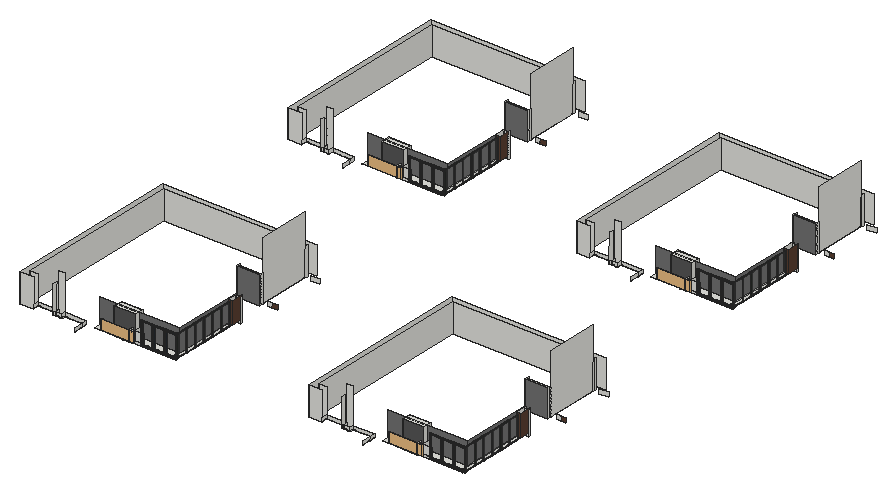
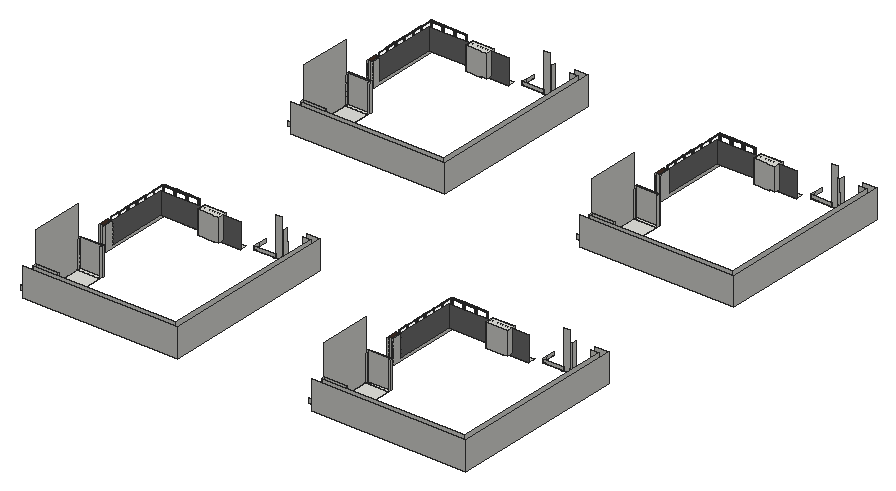
# SketchUp Ruby script. Lengths in inches.
U = 1.inch
M = Sketchup.active_model
def pt(a) = Geom::Point3d.new(a.map { |v| v * U })
def face(e, loops, mat)
  f = e.add_face(loops[0].map { |a| pt(a) })
  loops[1..].each { |l| e.add_face(l.map { |a| pt(a) }).erase! }
  f.material = f.back_material = mat if mat
  f
end
# faces: each face lists its corners as indices into pts; further lists are holes
def faces(e, pts, list, mat = nil) = list.each { |f| face(e, (f[0].is_a?(Array) ? f : [f]).map { |l| l.map { |i| pts[i] } }, mat) }
# xy, xz, yz: faces in a plane at the given z, y or x. An outline is a flat list of corners, or four numbers for a rectangle; further outlines are holes
def ring(l) = l.size == 4 ? [[l[0], l[1]], [l[2], l[1]], [l[2], l[3]], [l[0], l[3]]] : l.each_slice(2).to_a
def flat(e, list, mat, &to3) = list.each { |f| face(e, (f[0].is_a?(Array) ? f : [f]).map { |l| ring(l).map { |u, v| to3.(u, v) } }, mat) }
def xy(e, z, list, mat = nil) = flat(e, list, mat) { |x, y| [x, y, z] }
def xz(e, y, list, mat = nil) = flat(e, list, mat) { |x, z| [x, y, z] }
def yz(e, x, list, mat = nil) = flat(e, list, mat) { |y, z| [x, y, z] }
def lines(e, pts, list) = list.each { |a, b| e.add_line(pt(pts[a]), pt(pts[b])) }
# prism: a flat outline (further loops are holes) pulled along v
def prism(e, loops, v, mat = nil)
  f = face(e, loops, mat); d = Geom::Vector3d.new(v.map { |x| x * U })
  f.pushpull(f.normal.samedirection?(d) ? d.length : -d.length)
end
def box(e, o, s, mat = nil) = prism(e, [[o, [o[0] + s[0], o[1], o[2]], [o[0] + s[0], o[1] + s[1], o[2]], [o[0], o[1] + s[1], o[2]]]], [0, 0, s[2]], mat)
def at(x, y, z, deg = 0) = Geom::Transformation.translation(pt([x, y, z])) * Geom::Transformation.rotation(ORIGIN, Z_AXIS, deg.degrees)
def axes(o, x, y, z) = Geom::Transformation.new([*x, 0, *y, 0, *z, 0, *pt(o).to_a, 1])
def part(name) = M.definitions.add(name)
# library, detail: a bought-in or finely detailed component or shape, given as its bounding box
def library(name, o, s) = part(name).tap { |d| box(d.entities, o, s) }
def detail(e, o, s) = box(e.add_group.entities, o, s)
def put(e, d, t, mat = nil) = e.add_instance(d, t).tap { |i| i.material = mat if mat }
def group(e, t, mat = nil) = e.add_group.tap { |g| g.transformation = t; g.material = mat if mat }.entities
root = M.entities
M.materials.add("Glazing").color = [128, 128, 128]
M.materials["Glazing"].alpha = 0.05
M.materials.add("Powdercoating").color = [41, 44, 40]
M.materials.add("Wine2").color = [0, 0, 0]
M.materials["Wine2"].alpha = 0
M.materials.add("[0130_Gainsboro]").color = [39, 45, 50]
M.materials.add("[Color M05]").color = [114, 114, 114]
M.materials.add("[Color M06]").color = [86, 86, 86]
M.materials.add("[Granite Brown]").color = [89, 59, 61]
M.materials.add("[Granite Brown]1").color = [89, 63, 50]
c1 = library("Glass Railing",[0,0,0],[139.5,4.76,42])
c2 = part("Framed glazing panel")
xy(c2.entities,0,[[0,-0.98,43.07,0],[0,0,43.07,1.4]],"[0130_Gainsboro]")
xy(c2.entities,0.3,[[0.3,-1.43,42.77,-0.98]],"[0130_Gainsboro]")
xy(c2.entities,2.95,[[2.95,-1.43,40.12,-0.63],[2.95,-0.63,40.12,0],[2.95,0,40.12,0.64],[2.95,0.64,40.12,1.4]],"[0130_Gainsboro]")
xy(c2.entities,3.54,[[3.54,-0.63,39.53,0],[3.54,0,39.53,0.64]],"[0130_Gainsboro]")
xy(c2.entities,111.8125,[[3.54,-0.63,39.53,0],[3.54,0,39.53,0.64]],"[0130_Gainsboro]")
xy(c2.entities,112.4,[[2.95,-1.43,40.12,-0.63],[2.95,-0.63,40.12,0],[2.95,0,40.12,0.64],[2.95,0.64,40.12,1.4]],"[0130_Gainsboro]")
xy(c2.entities,115.05,[[0.3,-1.43,42.77,-0.98]],"[0130_Gainsboro]")
xy(c2.entities,115.35,[[0,-0.98,43.07,0],[0,0,43.07,1.4]],"[0130_Gainsboro]")
xz(c2.entities,-1.43,[[[0.3,0.3,42.77,115.05],[2.95,2.95,40.12,112.4]]],"[0130_Gainsboro]")
xz(c2.entities,-0.98,[[[0,0,43.07,115.35],[0.3,0.3,42.77,115.05]]],"[0130_Gainsboro]")
xz(c2.entities,-0.63,[[[2.95,2.95,40.12,112.4],[3.54,3.54,39.53,111.8125]]],"[0130_Gainsboro]")
xz(c2.entities,0,[[3.54,3.54,39.53,111.8125]],"Wine2")
xz(c2.entities,0,[[[0,0,43.07,115.35],[2.95,2.95,40.12,112.4]],[[2.95,2.95,40.12,112.4],[3.54,3.54,39.53,111.8125]]],"[0130_Gainsboro]")
xz(c2.entities,0.64,[[[2.95,2.95,40.12,112.4],[3.54,3.54,39.53,111.8125]]],"[0130_Gainsboro]")
xz(c2.entities,1.4,[[[0,0,43.07,115.35],[2.95,2.95,40.12,112.4]]],"[0130_Gainsboro]")
yz(c2.entities,0,[[-0.98,0,0,115.35],[0,0,1.4,115.35]],"[0130_Gainsboro]")
yz(c2.entities,0.3,[[-1.43,0.3,-0.98,115.05]],"[0130_Gainsboro]")
yz(c2.entities,2.95,[[-1.43,2.95,-0.63,112.4],[-0.63,2.95,0,112.4],[0,2.95,0.64,112.4],[0.64,2.95,1.4,112.4]],"[0130_Gainsboro]")
yz(c2.entities,3.54,[[-0.63,3.54,0,111.8125],[0,3.54,0.64,111.8125]],"[0130_Gainsboro]")
yz(c2.entities,39.53,[[-0.63,3.54,0,111.8125],[0,3.54,0.64,111.8125]],"[0130_Gainsboro]")
yz(c2.entities,40.12,[[-1.43,2.95,-0.63,112.4],[-0.63,2.95,0,112.4],[0,2.95,0.64,112.4],[0.64,2.95,1.4,112.4]],"[0130_Gainsboro]")
yz(c2.entities,42.77,[[-1.43,0.3,-0.98,115.05]],"[0130_Gainsboro]")
yz(c2.entities,43.07,[[-0.98,0,0,115.35],[0,0,1.4,115.35]],"[0130_Gainsboro]")
c3 = part("Glazed panel assembly")
put(c3.entities,c2,axes([90.57,1.43,0],[1.05148,0,0],[0,1,0],[0,0,1]))
put(c3.entities,c2,axes([0,1.43,0],[1.05148,0,0],[0,1,0],[0,0,1]))
put(c3.entities,c2,axes([45.29,1.43,0],[1.05148,0,0],[0,1,0],[0,0,1]))
c4 = part("Group\#15")
xy(c4.entities,0,[[0,-55.94,0.71,45.94]])
xy(c4.entities,0.2,[[0,-55.94,0.47,45.94],[0.47,45.94,0.71,46.42]])
xy(c4.entities,2.36,[[0.47,-55.94,0.71,46.42]])
xz(c4.entities,-55.94,[[0,0,0.71,0,0.71,2.36,0.47,2.36,0.47,0.2,0,0.2]])
xz(c4.entities,45.94,[[0,0,0.71,0.2]])
xz(c4.entities,46.42,[[0.47,0.2,0.71,2.36]])
yz(c4.entities,0,[[-55.94,0,45.94,0.2]])
yz(c4.entities,0.47,[[-55.94,0.2,46.42,2.36]])
yz(c4.entities,0.71,[[-55.94,0,45.94,0,45.94,0.2,46.42,0.2,46.42,2.36,-55.94,2.36]])
c5 = part("Group\#7")
xy(c5.entities,0,[[0,-59.09,0.71,45.94]])
xy(c5.entities,0.2,[[0,-59.09,0.47,45.94],[0.47,45.94,0.71,46.42]])
xy(c5.entities,2.36,[[0.47,-59.09,0.71,46.42]])
xz(c5.entities,-59.09,[[0,0,0.71,0,0.71,2.36,0.47,2.36,0.47,0.2,0,0.2]])
xz(c5.entities,45.94,[[0,0,0.71,0.2]])
xz(c5.entities,46.42,[[0.47,0.2,0.71,2.36]])
yz(c5.entities,0,[[-59.09,0,45.94,0.2]])
yz(c5.entities,0.47,[[-59.09,0.2,46.42,2.36]])
yz(c5.entities,0.71,[[-59.09,0,45.94,0,45.94,0.2,46.42,0.2,46.42,2.36,-59.09,2.36]])
c6 = part("Group\#16")
prism(c6.entities,[[[0.47,-56.18,0.2],[0,-56.18,0.2],[0,-56.18,0],[0.71,-56.18,0],[0.71,-56.18,2.36],[0.47,-56.18,2.36]]],[0,28.68,0])
c7 = part("Group\#10")
box(c7.entities,[-0.73,0,0],[27.99,0.55,102.05])
c8 = part("Group\#18")
xy(c8.entities,0,[[0.47,-56.18,0.47,-55.47,0,-55.47,0,-28.21,1.18,-28.21,1.18,-56.18]])
xy(c8.entities,0.2,[[0.71,-56.18,1.18,-28.21],[0,-55.47,0.47,-28.21],[0.47,-28.21,0.71,-27.74]])
xy(c8.entities,2.36,[[0.47,-56.18,0.71,-27.74]])
xz(c8.entities,-56.18,[[0.47,0,1.18,0,1.18,0.2,0.71,0.2,0.71,2.36,0.47,2.36]])
xz(c8.entities,-55.47,[[0,0,0.47,0.2]])
xz(c8.entities,-28.21,[[0,0,1.18,0.2]])
xz(c8.entities,-27.74,[[0.47,0.2,0.71,2.36]])
yz(c8.entities,0,[[-55.47,0,-28.21,0.2]])
yz(c8.entities,0.47,[[-56.18,0,-55.47,0.2],[-56.18,0.2,-27.74,2.36]])
yz(c8.entities,0.71,[[-56.18,0.2,-27.74,2.36]])
yz(c8.entities,1.18,[[-56.18,0,-28.21,0.2]])
c9 = part("Group\#34")
xy(c9.entities,0,[[-20.45,0,7.76,1.22]])
xy(c9.entities,0.06,[[-20.39,0.06,7.7,1.22]])
xy(c9.entities,0.47,[[-19.98,0,7.28,0.06]])
xy(c9.entities,101.89,[[-19.98,0,7.28,0.06]])
xy(c9.entities,102.3,[[-20.39,0.06,7.7,1.22]])
xy(c9.entities,102.36,[[-20.45,0,7.76,1.22]])
xz(c9.entities,0,[[[-20.45,0,7.76,102.36],[-19.98,0.47,7.28,101.89]]])
xz(c9.entities,0.06,[[[-20.39,0.06,7.7,102.3],[-19.98,0.47,7.28,101.89]]])
xz(c9.entities,1.22,[[[-20.45,0,7.76,102.36],[-20.39,0.06,7.7,102.3]]])
yz(c9.entities,-20.45,[[0,0,1.22,102.36]])
yz(c9.entities,-20.39,[[0.06,0.06,1.22,102.3]])
yz(c9.entities,-19.98,[[0,0.47,0.06,101.89]])
yz(c9.entities,7.28,[[0,0.47,0.06,101.89]])
yz(c9.entities,7.7,[[0.06,0.06,1.22,102.3]])
yz(c9.entities,7.76,[[0,0,1.22,102.36]])
c10 = part("Group\#6")
put(c10.entities,c4,axes([27.97,0,7.875],[1,0,0],[0,0,-1],[0,1,0]),"Powdercoating")
put(c10.entities,c5,axes([0.71,0,6.8],[-1,0,0],[0,0,-0.97687],[0,1,0]),"Powdercoating")
put(c10.entities,c6,axes([-27.5,0,-38.07],[0,0,-1],[-1,0,0],[0,1,0]),"Powdercoating")
put(c10.entities,c7,at(1.12,0.35,-38.39),"Glazing")
put(c10.entities,c8,axes([-27.5,0,63.35],[0,0,1],[-1,0,0],[0,1,0]),"Powdercoating")
put(c10.entities,c9,at(20.6875,1.0625,-38.54),"Powdercoating")
c11 = part("Sliding door assembly")
put(c11.entities,c10,at(-1.18,4.5,38.86))
g1 = group(c11.entities,at(84.74,4.5,38.86))
put(g1,c4,axes([-27.97,0,7.875],[-1,0,0],[0,0,-1],[0,1,0]),"Powdercoating")
put(g1,c5,axes([-0.71,0,6.8],[1,0,0],[0,0,-0.97687],[0,1,0]),"Powdercoating")
put(g1,c6,axes([27.5,0,-38.07],[0,0,-1],[1,0,0],[0,1,0]),"Powdercoating")
put(g1,c7,axes([-1.12,0.35,-38.39],[-1,0,0],[0,1,0],[0,0,1]),"Glazing")
put(g1,c8,axes([27.5,0,63.35],[0,0,1],[1,0,0],[0,1,0]),"Powdercoating")
put(g1,c9,axes([-20.6875,1.0625,-38.54],[-1,0,0],[0,1,0],[0,0,1]),"Powdercoating")
g2 = group(c11.entities,at(56.0625,4.5,38.86))
put(g2,c4,axes([-27.97,0,7.875],[-1,0,0],[0,0,-1],[0,1,0]),"Powdercoating")
put(g2,c6,axes([27.5,0,-38.07],[0,0,-1],[1,0,0],[0,1,0]),"Powdercoating")
put(g2,c7,axes([-1.12,0.35,-38.39],[-1,0,0],[0,1,0],[0,0,1]),"Glazing")
put(g2,c8,axes([27.5,0,63.35],[0,0,1],[1,0,0],[0,1,0]),"Powdercoating")
put(g2,c9,axes([-20.6875,1.0625,-38.54],[-1,0,0],[0,1,0],[0,0,1]),"Powdercoating")
g3 = group(g2,at(-0.71,0,6.8),"Powdercoating")
xy(g3,-45.34,[[0.47,0.2,0.71,2.36]])
xy(g3,-44.88,[[0,0,0.71,0.2]])
xy(g3,57.73,[[0,0,0.71,0,0.71,2.36,0.47,2.36,0.47,0.2,0,0.2]])
xz(g3,0,[[0,-44.88,0.71,57.73]])
xz(g3,0.2,[[0.47,-45.34,0.71,-44.88],[0,-44.88,0.47,57.73]])
xz(g3,2.36,[[0.47,-45.34,0.71,57.73]])
yz(g3,0,[[0,-44.88,0.2,57.73]])
yz(g3,0.47,[[0.2,-45.34,2.36,57.73]])
yz(g3,0.71,[[0.2,-45.34,2.36,-45.34,2.36,57.73,0,57.73,0,-44.88,0.2,-44.88]])
put(c11.entities,c10,axes([-33.94,4.5,38.86],[1.14218,0,0],[0,1,0],[0,0,1]))
c12 = part("sliding door")
put(c12.entities,c11,at(0,-4.5,-0.08))
xy(root,1644,[[679.51,1822.9375,709.01,1824.0625],[709.01,1822.9375,709.36,1827.125],[1897.7,1822.9375,1927.2,1824.0625],[1927.2,1822.9375,1927.54,1827.125],[557.88,1824.0625,679.51,1824.0625,679.51,1827.125,709.01,1827.125,709.01,1851.6875,557.88,1851.6875],
  [679.51,1824.0625,709.01,1827.125],[1776.07,1824.0625,1897.7,1824.0625,1897.7,1827.125,1927.2,1827.125,1927.2,1851.6875,1776.07,1851.6875],[1897.7,1824.0625,1927.2,1827.125],[894.3125,2148.625,913.875,2156.01],[2112.5,2148.625,2132.0625,2156.01],
  [795.3125,2295.875,890.875,2518.89],[2013.5,2295.875,2109.0625,2518.89],[679.51,3237.625,709.01,3238.75],[709.01,3237.625,709.36,3241.8125],[1897.7,3237.625,1927.2,3238.75],
  [1927.2,3237.625,1927.54,3241.8125],[557.88,3238.75,679.51,3238.75,679.51,3241.8125,709.01,3241.8125,709.01,3266.375,557.88,3266.375],[679.51,3238.75,709.01,3241.8125],[1776.07,3238.75,1897.7,3238.75,1897.7,3241.8125,1927.2,3241.8125,1927.2,3266.375,1776.07,3266.375],[1897.7,3238.75,1927.2,3241.8125],
  [894.3125,3563.3125,913.875,3570.7],[2112.5,3563.3125,2132.0625,3570.7],[795.3125,3710.5625,890.875,3933.57],[2013.5,3710.5625,2109.0625,3933.57]])
xy(root,1644,[[557.4,1822.9375,557.88,1824.0625],[1775.59,1822.9375,1776.07,1824.0625],[557.4,3237.625,557.88,3238.75],[1775.59,3237.625,1776.07,3238.75]],"[Granite Brown]")
xy(root,1645.75,[[795.3125,2278.25,890.875,2284.4375],[2013.5,2278.25,2109.0625,2284.4375],[795.3125,2284.4375,890.875,2295.875],[2013.5,2284.4375,2109.0625,2295.875],[795.3125,2295.875,890.875,2517.14],
  [2013.5,2295.875,2109.0625,2517.14],[795.3125,2517.14,890.875,2518.89],[2013.5,2517.14,2109.0625,2518.89],[795.3125,3692.9375,890.875,3699.125],[2013.5,3692.9375,2109.0625,3699.125],
  [795.3125,3699.125,890.875,3710.5625],[2013.5,3699.125,2109.0625,3710.5625],[795.3125,3710.5625,890.875,3931.82],[2013.5,3710.5625,2109.0625,3931.82],[795.3125,3931.82,890.875,3933.57],
  [2013.5,3931.82,2109.0625,3933.57]])
xy(root,1650.875,[[589.79,1814.25,709.36,1822.9375],[1807.98,1814.25,1927.54,1822.9375],[589.79,3228.9375,709.36,3237.625],[1807.98,3228.9375,1927.54,3237.625]])
xy(root,1650.88,[[652.3,1835.1875,668.6,1873.375],[668.6,1835.1875,670.29,1873.375],[670.29,1835.1875,721.4,1873.375],[1870.49,1835.1875,1886.79,1873.375],[1886.79,1835.1875,1888.48,1873.375],
  [1888.48,1835.1875,1939.59,1873.375],[652.3,3249.875,668.6,3288.0625],[668.6,3249.875,670.29,3288.0625],[670.29,3249.875,721.4,3288.0625],[1870.49,3249.875,1886.79,3288.0625],
  [1886.79,3249.875,1888.48,3288.0625],[1888.48,3249.875,1939.59,3288.0625]])
xy(root,1651.2,[[631.46,1835.1875,652.3,1873.375],[1849.65,1835.1875,1870.49,1873.375],[631.46,3249.875,652.3,3288.0625],[1849.65,3249.875,1870.49,3288.0625]])
xy(root,1656.6875,[[764.59,1814.25,913.875,1814.25,913.875,2107.9375,894.3125,2107.9375,894.3125,1822.9375,764.59,1822.9375],[1982.78,1814.25,2132.0625,1814.25,2132.0625,2107.9375,2112.5,2107.9375,2112.5,1822.9375,1982.78,1822.9375],[727.9,1822.9375,890.875,1851.6875],[890.875,1822.9375,894.3125,1851.6875],[1946.09,1822.9375,2109.0625,1851.6875],
  [2109.0625,1822.9375,2112.5,1851.6875],[764.59,3228.9375,913.875,3228.9375,913.875,3522.625,894.3125,3522.625,894.3125,3237.625,764.59,3237.625],[1982.78,3228.9375,2132.0625,3228.9375,2132.0625,3522.625,2112.5,3522.625,2112.5,3237.625,1982.78,3237.625],[727.9,3237.625,890.875,3266.375],[890.875,3237.625,894.3125,3266.375],
  [1946.09,3237.625,2109.0625,3266.375],[2109.0625,3237.625,2112.5,3266.375]])
xy(root,1749.01,[[631.46,1835.1875,721.4,1873.375],[1849.65,1835.1875,1939.59,1873.375],[631.46,3249.875,721.4,3288.0625],[1849.65,3249.875,1939.59,3288.0625]])
xz(root,1799.9375,[[262.875,1644,319.53,1764],[1481.0625,1644,1537.72,1764]])
xz(root,1806.5625,[[406.84,1644,431.33,1644.0625],[1625.03,1644,1649.52,1644.0625],[406.84,1644.0625,431.33,1644.125],[1625.03,1644.0625,1649.52,1644.125],[406.84,1644.125,406.84,1659.3125,396.11,1659.37,396.03,1644.18],
  [406.84,1644.125,406.92,1659.3125,406.84,1659.3125],[406.84,1644.125,431.33,1644.125,431.33,1659.3125,406.92,1659.3125],[1625.03,1644.125,1625.03,1659.3125,1614.29,1659.37,1614.22,1644.18],[1625.03,1644.125,1625.11,1659.3125,1625.03,1659.3125],[1625.03,1644.125,1649.52,1644.125,1649.52,1659.3125,1625.11,1659.3125]])
xz(root,1822.9375,[[285.875,1644,319.53,1764],[319.53,1644,406.84,1644.0625],[406.84,1644,406.84,1644.125,407.44,1764,407.65,1805.3125,407.44,1805.3125,407.44,1807.33,431.33,1807.33,431.33,1644],[431.33,1644,523.04,1644.0625],[679.51,1644,709.01,1650.875],
  [709.01,1644,709.36,1650.875],[709.36,1644,890.875,1644,890.875,1656.6875,727.9,1656.6875,727.9,1693.1875,709.36,1693.1875],[890.875,1644,894.3125,1656.6875],[1504.0625,1644,1537.72,1764],[1537.72,1644,1625.03,1644.0625],
  [1625.03,1644,1625.03,1644.125,1625.63,1764,1625.84,1805.3125,1625.63,1805.3125,1625.63,1807.33,1649.52,1807.33,1649.52,1644],[1649.52,1644,1741.23,1644.0625],[1897.7,1644,1927.2,1650.875],[1927.2,1644,1927.54,1650.875],[1927.54,1644,2109.0625,1644,2109.0625,1656.6875,1946.09,1656.6875,1946.09,1693.1875,1927.54,1693.1875],
  [2109.0625,1644,2112.5,1656.6875],[319.53,1644.0625,406.84,1644.125],[431.33,1644.0625,523.04,1644.125],[1537.72,1644.0625,1625.03,1644.125],[1649.52,1644.0625,1741.23,1644.125],
  [319.53,1644.125,406.84,1644.125,396.03,1644.18,396.11,1659.3125,319.53,1659.3125],[406.84,1644.125,396.03,1644.18,396.11,1659.3125,406.84,1659.3125],[406.84,1644.125,407.44,1764,396.63,1764,396.11,1659.3125,406.84,1659.3125],[431.33,1644.125,523.04,1659.3125],[1537.72,1644.125,1625.03,1644.125,1614.22,1644.18,1614.29,1659.3125,1537.72,1659.3125],
  [1625.03,1644.125,1614.22,1644.18,1614.29,1659.3125,1625.03,1659.3125],[1625.03,1644.125,1625.63,1764,1614.82,1764,1614.29,1659.3125,1625.03,1659.3125],[1649.52,1644.125,1741.23,1659.3125],[709.01,1650.875,709.36,1693.1875],[1927.2,1650.875,1927.54,1693.1875],
  [727.9,1656.6875,764.59,1693.1875],[1946.09,1656.6875,1982.78,1693.1875]])
xz(root,1835.1875,[[652.3,1650.88,721.4,1650.88,721.4,1749.01,631.46,1749.01,631.46,1651.2,652.3,1651.2],[1870.49,1650.88,1939.59,1650.88,1939.59,1749.01,1849.65,1749.01,1849.65,1651.2,1870.49,1651.2]],"[Color M06]")
xz(root,1851.6875,[[557.88,1644,709.01,1644,709.01,1693.1875,727.9,1693.1875,727.9,1656.6875,894.3125,1656.6875,894.3125,1749.375,557.88,1749.375],[1776.07,1644,1927.2,1644,1927.2,1693.1875,1946.09,1693.1875,1946.09,1656.6875,2112.5,1656.6875,2112.5,1749.375,1776.07,1749.375]],"[Color M05]")
xz(root,1873.375,[[652.3,1650.88,652.3,1651.2,631.46,1651.2,631.46,1749.01,721.4,1749.01,721.4,1650.88],[1870.49,1650.88,1870.49,1651.2,1849.65,1651.2,1849.65,1749.01,1939.59,1749.01,1939.59,1650.88]])
xz(root,2107.9375,[[894.3125,1656.6875,913.875,1747],[2112.5,1656.6875,2132.0625,1747]],"[Granite Brown]1")
xz(root,2148.625,[[894.3125,1644,913.875,1747],[2112.5,1644,2132.0625,1747]])
xz(root,2156.01,[[894.3125,1644,913.875,1661.36],[2112.5,1644,2132.0625,1661.36]])
xz(root,2278.25,[[795.3125,1645.75,890.875,1764],[2013.5,1645.75,2109.0625,1764]],"[Color M05]")
xz(root,2284.4375,[[795.3125,1645.75,890.875,1764],[2013.5,1645.75,2109.0625,1764]])
xz(root,2295.875,[[795.3125,1644,890.875,1645.75],[913.875,1644,930.75,1663.0625],[2013.5,1644,2109.0625,1645.75],[2132.0625,1644,2148.9375,1663.0625]])
xz(root,2295.875,[[930.75,1644,954.6875,1663.0625],[2148.9375,1644,2172.875,1663.0625]],"[Granite Brown]1")
xz(root,2517.14,[[795.3125,1645.75,890.875,1764],[2013.5,1645.75,2109.0625,1764]])
xz(root,2518.89,[[795.3125,1644,890.875,1645.75],[913.875,1644,954.6875,1663.0625],[2013.5,1644,2109.0625,1645.75],[2132.0625,1644,2172.875,1663.0625],[795.3125,1645.75,890.875,1764],
  [2013.5,1645.75,2109.0625,1764]])
xz(root,2531.375,[[285.875,1644,890.875,1764],[1504.0625,1644,2109.0625,1764]])
xz(root,2554.375,[[262.875,1644,913.875,1764],[1481.0625,1644,2132.0625,1764]])
xz(root,3214.625,[[262.875,1644,319.53,1764],[1481.0625,1644,1537.72,1764]])
xz(root,3221.25,[[406.84,1644,431.33,1644.0625],[1625.03,1644,1649.52,1644.0625],[406.84,1644.0625,431.33,1644.125],[1625.03,1644.0625,1649.52,1644.125],[406.84,1644.125,406.84,1659.3125,396.11,1659.37,396.03,1644.18],
  [406.84,1644.125,406.92,1659.3125,406.84,1659.3125],[406.84,1644.125,431.33,1644.125,431.33,1659.3125,406.92,1659.3125],[1625.03,1644.125,1625.03,1659.3125,1614.29,1659.37,1614.22,1644.18],[1625.03,1644.125,1625.11,1659.3125,1625.03,1659.3125],[1625.03,1644.125,1649.52,1644.125,1649.52,1659.3125,1625.11,1659.3125]])
xz(root,3237.625,[[285.875,1644,319.53,1764],[319.53,1644,406.84,1644.0625],[406.84,1644,406.84,1644.125,407.44,1764,407.65,1805.3125,407.44,1805.3125,407.44,1807.33,431.33,1807.33,431.33,1644],[431.33,1644,523.04,1644.0625],[679.51,1644,709.01,1650.875],
  [709.01,1644,709.36,1650.875],[709.36,1644,890.875,1644,890.875,1656.6875,727.9,1656.6875,727.9,1693.1875,709.36,1693.1875],[890.875,1644,894.3125,1656.6875],[1504.0625,1644,1537.72,1764],[1537.72,1644,1625.03,1644.0625],
  [1625.03,1644,1625.03,1644.125,1625.63,1764,1625.84,1805.3125,1625.63,1805.3125,1625.63,1807.33,1649.52,1807.33,1649.52,1644],[1649.52,1644,1741.23,1644.0625],[1897.7,1644,1927.2,1650.875],[1927.2,1644,1927.54,1650.875],[1927.54,1644,2109.0625,1644,2109.0625,1656.6875,1946.09,1656.6875,1946.09,1693.1875,1927.54,1693.1875],
  [2109.0625,1644,2112.5,1656.6875],[319.53,1644.0625,406.84,1644.125],[431.33,1644.0625,523.04,1644.125],[1537.72,1644.0625,1625.03,1644.125],[1649.52,1644.0625,1741.23,1644.125],
  [319.53,1644.125,406.84,1644.125,396.03,1644.18,396.11,1659.3125,319.53,1659.3125],[406.84,1644.125,396.03,1644.18,396.11,1659.3125,406.84,1659.3125],[406.84,1644.125,407.44,1764,396.63,1764,396.11,1659.3125,406.84,1659.3125],[431.33,1644.125,523.04,1659.3125],[1537.72,1644.125,1625.03,1644.125,1614.22,1644.18,1614.29,1659.3125,1537.72,1659.3125],
  [1625.03,1644.125,1614.22,1644.18,1614.29,1659.3125,1625.03,1659.3125],[1625.03,1644.125,1625.63,1764,1614.82,1764,1614.29,1659.3125,1625.03,1659.3125],[1649.52,1644.125,1741.23,1659.3125],[709.01,1650.875,709.36,1693.1875],[1927.2,1650.875,1927.54,1693.1875],
  [727.9,1656.6875,764.59,1693.1875],[1946.09,1656.6875,1982.78,1693.1875]])
xz(root,3249.875,[[652.3,1650.88,721.4,1650.88,721.4,1749.01,631.46,1749.01,631.46,1651.2,652.3,1651.2],[1870.49,1650.88,1939.59,1650.88,1939.59,1749.01,1849.65,1749.01,1849.65,1651.2,1870.49,1651.2]],"[Color M06]")
xz(root,3266.375,[[557.88,1644,709.01,1644,709.01,1693.1875,727.9,1693.1875,727.9,1656.6875,894.3125,1656.6875,894.3125,1749.375,557.88,1749.375],[1776.07,1644,1927.2,1644,1927.2,1693.1875,1946.09,1693.1875,1946.09,1656.6875,2112.5,1656.6875,2112.5,1749.375,1776.07,1749.375]],"[Color M05]")
xz(root,3288.0625,[[652.3,1650.88,652.3,1651.2,631.46,1651.2,631.46,1749.01,721.4,1749.01,721.4,1650.88],[1870.49,1650.88,1870.49,1651.2,1849.65,1651.2,1849.65,1749.01,1939.59,1749.01,1939.59,1650.88]])
xz(root,3522.625,[[894.3125,1656.6875,913.875,1747],[2112.5,1656.6875,2132.0625,1747]],"[Granite Brown]1")
xz(root,3563.3125,[[894.3125,1644,913.875,1747],[2112.5,1644,2132.0625,1747]])
xz(root,3570.7,[[894.3125,1644,913.875,1661.36],[2112.5,1644,2132.0625,1661.36]])
xz(root,3692.9375,[[795.3125,1645.75,890.875,1764],[2013.5,1645.75,2109.0625,1764]],"[Color M05]")
xz(root,3699.125,[[795.3125,1645.75,890.875,1764],[2013.5,1645.75,2109.0625,1764]])
xz(root,3710.5625,[[795.3125,1644,890.875,1645.75],[913.875,1644,930.75,1663.0625],[2013.5,1644,2109.0625,1645.75],[2132.0625,1644,2148.9375,1663.0625]])
xz(root,3710.5625,[[930.75,1644,954.6875,1663.0625],[2148.9375,1644,2172.875,1663.0625]],"[Granite Brown]1")
xz(root,3931.82,[[795.3125,1645.75,890.875,1764],[2013.5,1645.75,2109.0625,1764]])
xz(root,3933.57,[[795.3125,1644,890.875,1645.75],[913.875,1644,954.6875,1663.0625],[2013.5,1644,2109.0625,1645.75],[2132.0625,1644,2172.875,1663.0625],[795.3125,1645.75,890.875,1764],
  [2013.5,1645.75,2109.0625,1764]])
xz(root,3946.0625,[[285.875,1644,890.875,1764],[1504.0625,1644,2109.0625,1764]])
xz(root,3969.0625,[[262.875,1644,913.875,1764],[1481.0625,1644,2132.0625,1764]])
yz(root,262.875,[[1799.9375,1644,2554.375,1764],[3214.625,1644,3969.0625,1764]])
yz(root,285.875,[[1822.9375,1644,2531.375,1764],[3237.625,1644,3946.0625,1764]])
yz(root,319.53,[[1799.9375,1644,1822.9375,1644.0625],[3214.625,1644,3237.625,1644.0625],[1799.9375,1644.0625,1822.9375,1644.125],[3214.625,1644.0625,3237.625,1644.125],[1799.9375,1644.125,1822.9375,1659.3125],
  [3214.625,1644.125,3237.625,1659.3125]])
yz(root,406.84,[[1806.5625,1644,1822.9375,1644.0625],[3221.25,1644,3237.625,1644.0625],[1806.5625,1644.0625,1822.9375,1644.125],[3221.25,1644.0625,3237.625,1644.125],[1806.5625,1644.125,1822.9375,1659.3125],
  [3221.25,1644.125,3237.625,1659.3125]])
yz(root,431.33,[[1806.5625,1644,1822.9375,1644.0625],[3221.25,1644,3237.625,1644.0625],[1806.5625,1644.0625,1822.9375,1644.125],[3221.25,1644.0625,3237.625,1644.125],[1806.5625,1644.125,1822.9375,1659.3125],
  [3221.25,1644.125,3237.625,1659.3125]])
yz(root,523.04,[[1763.25,1644,1799.9375,1644.0625],[1799.9375,1644,1822.9375,1644.0625],[3177.9375,1644,3214.625,1644.0625],[3214.625,1644,3237.625,1644.0625],[1763.25,1644.0625,1799.9375,1644.125],
  [1799.9375,1644.0625,1822.9375,1644.125],[3177.9375,1644.0625,3214.625,1644.125],[3214.625,1644.0625,3237.625,1644.125],[1763.25,1644.125,1799.9375,1659.3125],[1799.9375,1644.125,1822.9375,1659.3125],
  [3177.9375,1644.125,3214.625,1659.3125],[3214.625,1644.125,3237.625,1659.3125]])
yz(root,631.46,[[1835.1875,1651.2,1873.375,1749.01],[3249.875,1651.2,3288.0625,1749.01]])
yz(root,652.3,[[1835.1875,1650.88,1873.375,1651.2],[3249.875,1650.88,3288.0625,1651.2]])
yz(root,709.01,[[1822.9375,1644,1851.6875,1693.1875],[3237.625,1644,3266.375,1693.1875]])
yz(root,709.36,[[1814.25,1650.875,1822.9375,1693.1875],[3228.9375,1650.875,3237.625,1693.1875]])
yz(root,721.4,[[1835.1875,1650.88,1873.375,1749.01],[3249.875,1650.88,3288.0625,1749.01]])
yz(root,727.9,[[1822.9375,1656.6875,1851.6875,1693.1875],[3237.625,1656.6875,3266.375,1693.1875]])
yz(root,764.59,[[1814.25,1656.6875,1822.9375,1693.1875],[3228.9375,1656.6875,3237.625,1693.1875]])
yz(root,795.3125,[[2295.875,1644,2518.89,1645.75],[3710.5625,1644,3933.57,1645.75],[2278.25,1645.75,2284.4375,1764],[2284.4375,1645.75,2295.875,1764],[2517.14,1645.75,2518.89,1764],
  [3692.9375,1645.75,3699.125,1764],[3699.125,1645.75,3710.5625,1764],[3931.82,1645.75,3933.57,1764]])
yz(root,890.875,[[2295.875,1644,2518.89,1645.75],[2518.89,1644,2531.375,1764],[3710.5625,1644,3933.57,1645.75],[3933.57,1644,3946.0625,1764],[2278.25,1645.75,2284.4375,1764],
  [2284.4375,1645.75,2295.875,1764],[2295.875,1645.75,2517.14,1895.25],[2517.14,1645.75,2518.89,1764],[3692.9375,1645.75,3699.125,1764],[3699.125,1645.75,3710.5625,1764],
  [3710.5625,1645.75,3931.82,1895.25],[3931.82,1645.75,3933.57,1764]])
yz(root,894.3125,[[1822.9375,1644,2148.625,1644,2148.625,1747,2107.9375,1747,2107.9375,1656.6875,1822.9375,1656.6875],[2148.83,1644,2156.01,1747.04],[3237.625,1644,3563.3125,1644,3563.3125,1747,3522.625,1747,3522.625,1656.6875,3237.625,1656.6875],[3563.51,1644,3570.7,1747.04]])
yz(root,894.3125,[[2148.625,1644,2148.83,1644,2148.83,1749.375,1851.6875,1749.375,1851.6875,1656.6875,2107.9375,1656.6875,2107.9375,1747,2148.625,1747],[3563.3125,1644,3563.51,1644,3563.51,1749.375,3266.375,1749.375,3266.375,1656.6875,3522.625,1656.6875,3522.625,1747,3563.3125,1747]],"[Color M05]")
yz(root,913.875,[[2148.83,1644,2156.01,1747.04],[3563.51,1644,3570.7,1747.04]])
yz(root,913.875,[[2107.9375,1656.6875,2148.625,1747],[3522.625,1656.6875,3563.3125,1747]],"[Granite Brown]1")
yz(root,1481.0625,[[1799.9375,1644,2554.375,1764],[3214.625,1644,3969.0625,1764]])
yz(root,1504.0625,[[1822.9375,1644,2531.375,1764],[3237.625,1644,3946.0625,1764]])
yz(root,1537.72,[[1799.9375,1644,1822.9375,1644.0625],[3214.625,1644,3237.625,1644.0625],[1799.9375,1644.0625,1822.9375,1644.125],[3214.625,1644.0625,3237.625,1644.125],[1799.9375,1644.125,1822.9375,1659.3125],
  [3214.625,1644.125,3237.625,1659.3125]])
yz(root,1625.03,[[1806.5625,1644,1822.9375,1644.0625],[3221.25,1644,3237.625,1644.0625],[1806.5625,1644.0625,1822.9375,1644.125],[3221.25,1644.0625,3237.625,1644.125],[1806.5625,1644.125,1822.9375,1659.3125],
  [3221.25,1644.125,3237.625,1659.3125]])
yz(root,1649.52,[[1806.5625,1644,1822.9375,1644.0625],[3221.25,1644,3237.625,1644.0625],[1806.5625,1644.0625,1822.9375,1644.125],[3221.25,1644.0625,3237.625,1644.125],[1806.5625,1644.125,1822.9375,1659.3125],
  [3221.25,1644.125,3237.625,1659.3125]])
yz(root,1741.23,[[1763.25,1644,1799.9375,1644.0625],[1799.9375,1644,1822.9375,1644.0625],[3177.9375,1644,3214.625,1644.0625],[3214.625,1644,3237.625,1644.0625],[1763.25,1644.0625,1799.9375,1644.125],
  [1799.9375,1644.0625,1822.9375,1644.125],[3177.9375,1644.0625,3214.625,1644.125],[3214.625,1644.0625,3237.625,1644.125],[1763.25,1644.125,1799.9375,1659.3125],[1799.9375,1644.125,1822.9375,1659.3125],
  [3177.9375,1644.125,3214.625,1659.3125],[3214.625,1644.125,3237.625,1659.3125]])
yz(root,1849.65,[[1835.1875,1651.2,1873.375,1749.01],[3249.875,1651.2,3288.0625,1749.01]])
yz(root,1870.49,[[1835.1875,1650.88,1873.375,1651.2],[3249.875,1650.88,3288.0625,1651.2]])
yz(root,1927.2,[[1822.9375,1644,1851.6875,1693.1875],[3237.625,1644,3266.375,1693.1875]])
yz(root,1927.54,[[1814.25,1650.875,1822.9375,1693.1875],[3228.9375,1650.875,3237.625,1693.1875]])
yz(root,1939.59,[[1835.1875,1650.88,1873.375,1749.01],[3249.875,1650.88,3288.0625,1749.01]])
yz(root,1946.09,[[1822.9375,1656.6875,1851.6875,1693.1875],[3237.625,1656.6875,3266.375,1693.1875]])
yz(root,1982.78,[[1814.25,1656.6875,1822.9375,1693.1875],[3228.9375,1656.6875,3237.625,1693.1875]])
yz(root,2013.5,[[2295.875,1644,2518.89,1645.75],[3710.5625,1644,3933.57,1645.75],[2278.25,1645.75,2284.4375,1764],[2284.4375,1645.75,2295.875,1764],[2517.14,1645.75,2518.89,1764],
  [3692.9375,1645.75,3699.125,1764],[3699.125,1645.75,3710.5625,1764],[3931.82,1645.75,3933.57,1764]])
yz(root,2109.0625,[[2295.875,1644,2518.89,1645.75],[2518.89,1644,2531.375,1764],[3710.5625,1644,3933.57,1645.75],[3933.57,1644,3946.0625,1764],[2278.25,1645.75,2284.4375,1764],
  [2284.4375,1645.75,2295.875,1764],[2295.875,1645.75,2517.14,1895.25],[2517.14,1645.75,2518.89,1764],[3692.9375,1645.75,3699.125,1764],[3699.125,1645.75,3710.5625,1764],
  [3710.5625,1645.75,3931.82,1895.25],[3931.82,1645.75,3933.57,1764]])
yz(root,2112.5,[[1822.9375,1644,2148.625,1644,2148.625,1747,2107.9375,1747,2107.9375,1656.6875,1822.9375,1656.6875],[2148.83,1644,2156.01,1747.04],[3237.625,1644,3563.3125,1644,3563.3125,1747,3522.625,1747,3522.625,1656.6875,3237.625,1656.6875],[3563.51,1644,3570.7,1747.04]])
yz(root,2112.5,[[2148.625,1644,2148.83,1644,2148.83,1749.375,1851.6875,1749.375,1851.6875,1656.6875,2107.9375,1656.6875,2107.9375,1747,2148.625,1747],[3563.3125,1644,3563.51,1644,3563.51,1749.375,3266.375,1749.375,3266.375,1656.6875,3522.625,1656.6875,3522.625,1747,3563.3125,1747]],"[Color M05]")
yz(root,2132.0625,[[2148.83,1644,2156.01,1747.04],[3563.51,1644,3570.7,1747.04]])
yz(root,2132.0625,[[2107.9375,1656.6875,2148.625,1747],[3522.625,1656.6875,3563.3125,1747]],"[Granite Brown]1")
p = [[406.84,1822.9375,1644.125],[406.84,1806.5625,1644.125],[396.03,1806.5625,1644.18],[396.03,1822.9375,1644.18],[1625.03,1822.9375,1644.125],[1625.03,1806.5625,1644.125],
  [1614.22,1806.5625,1644.18],[1614.22,1822.9375,1644.18],[406.84,3237.625,1644.125],[406.84,3221.25,1644.125],[396.03,3221.25,1644.18],[396.03,3237.625,1644.18],
  [1625.03,3237.625,1644.125],[1625.03,3221.25,1644.125],[1614.22,3221.25,1644.18],[1614.22,3237.625,1644.18],[396.63,1822.9375,1764.05],[396.63,1822.9375,1764],
  [396.11,1822.9375,1659.3125],[396.11,1806.5625,1659.37],[396.63,1806.5625,1764.05],[1614.82,1822.9375,1764.05],[1614.82,1822.9375,1764],[1614.29,1822.9375,1659.3125],
  [1614.29,1806.5625,1659.37],[1614.82,1806.5625,1764.05],[396.63,3237.625,1764.05],[396.63,3237.625,1764],[396.11,3237.625,1659.3125],[396.11,3221.25,1659.37],
  [396.63,3221.25,1764.05],[1614.82,3237.625,1764.05],[1614.82,3237.625,1764],[1614.29,3237.625,1659.3125],[1614.29,3221.25,1659.37],[1614.82,3221.25,1764.05]]
faces(root,p,[[0,1,2,3],[4,5,6,7],[8,9,10,11],[12,13,14,15],[16,17,18,3,2,19,20],[21,22,23,7,6,24,25],[26,27,28,11,10,29,30],[31,32,33,15,14,34,35]])
put(root,c1,at(1807.98,1814.25,1650.875),"[Granite Brown]")
put(root,c1,at(589.79,1814.25,1650.875),"[Granite Brown]")
put(root,c1,at(1807.98,3228.9375,1650.875),"[Granite Brown]")
put(root,c1,at(589.79,3228.9375,1650.875),"[Granite Brown]")
put(root,c3,axes([1979.67,1814.25,1653.73],[1.12,0,0],[0,1,0],[0,0,0.8291]),"[Color M06]")
put(root,c3,axes([761.48,1814.25,1653.73],[1.12,0,0],[0,1,0],[0,0,0.8291]),"[Color M06]")
put(root,c3,axes([1979.67,3228.9375,1653.73],[1.12,0,0],[0,1,0],[0,0,0.8291]),"[Color M06]")
put(root,c3,axes([761.48,3228.9375,1653.73],[1.12,0,0],[0,1,0],[0,0,0.8291]),"[Color M06]")
put(root,c12,axes([2132.0625,1867.65,1656.6875],[0,1.55,0],[-1,0,0],[0,0,0.8972]),"[Color M06]")
put(root,c12,axes([913.875,1867.65,1656.6875],[0,1.55,0],[-1,0,0],[0,0,0.8972]),"[Color M06]")
put(root,c12,axes([2132.0625,3282.33,1656.6875],[0,1.55,0],[-1,0,0],[0,0,0.8972]),"[Color M06]")
put(root,c12,axes([913.875,3282.33,1656.6875],[0,1.55,0],[-1,0,0],[0,0,0.8972]),"[Color M06]")
put(root,c12,axes([2132.0625,1961.78,1656.6875],[0,1.55,0],[-1,0,0],[0,0,0.8972]))
put(root,c12,axes([913.875,1961.78,1656.6875],[0,1.55,0],[-1,0,0],[0,0,0.8972]))
put(root,c12,axes([2132.0625,3376.47,1656.6875],[0,1.55,0],[-1,0,0],[0,0,0.8972]))
put(root,c12,axes([913.875,3376.47,1656.6875],[0,1.55,0],[-1,0,0],[0,0,0.8972]))
